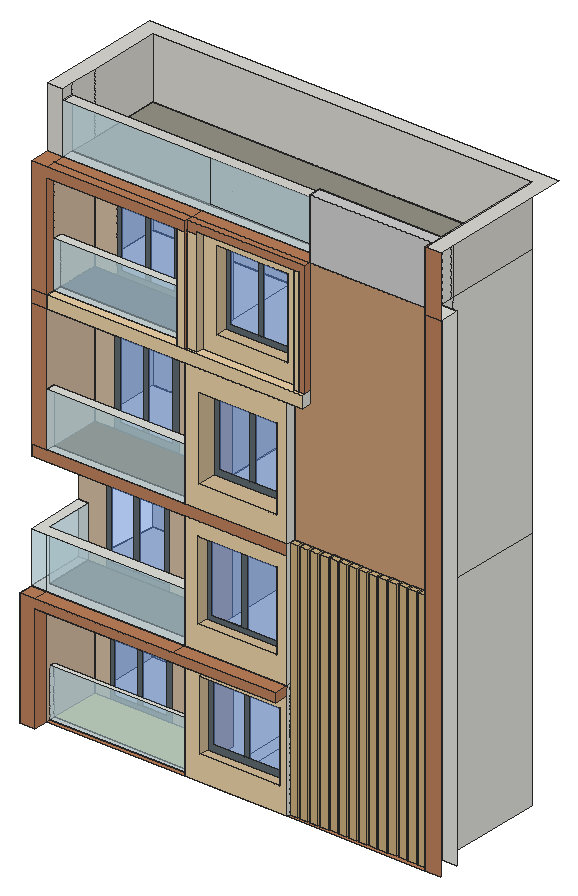
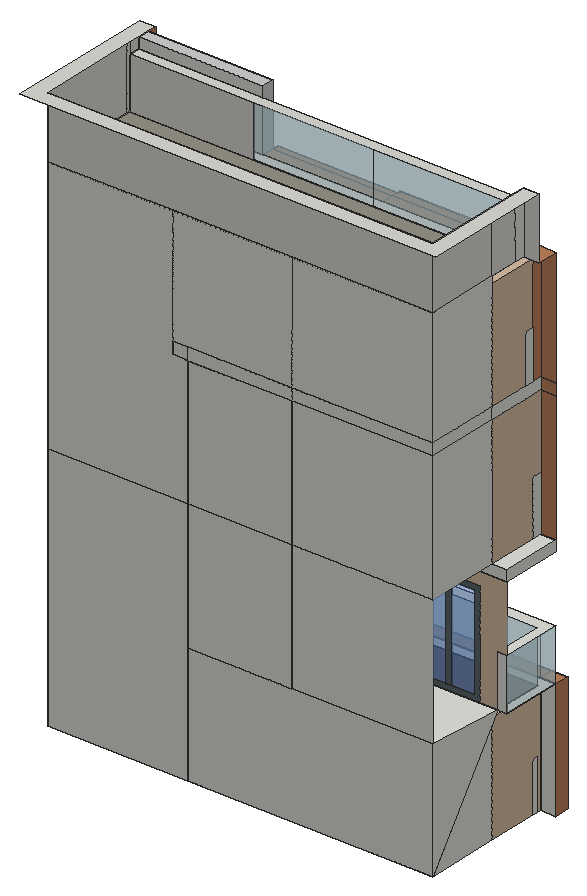
# SketchUp Ruby script. Lengths in inches.
U = 1.inch
M = Sketchup.active_model
def pt(a) = Geom::Point3d.new(a.map { |v| v * U })
def face(e, loops, mat)
  f = e.add_face(loops[0].map { |a| pt(a) })
  loops[1..].each { |l| e.add_face(l.map { |a| pt(a) }).erase! }
  f.material = f.back_material = mat if mat
  f
end
# faces: each face lists its corners as indices into pts; further lists are holes
def faces(e, pts, list, mat = nil) = list.each { |f| face(e, (f[0].is_a?(Array) ? f : [f]).map { |l| l.map { |i| pts[i] } }, mat) }
# xy, xz, yz: faces in a plane at the given z, y or x. An outline is a flat list of corners, or four numbers for a rectangle; further outlines are holes
def ring(l) = l.size == 4 ? [[l[0], l[1]], [l[2], l[1]], [l[2], l[3]], [l[0], l[3]]] : l.each_slice(2).to_a
def flat(e, list, mat, &to3) = list.each { |f| face(e, (f[0].is_a?(Array) ? f : [f]).map { |l| ring(l).map { |u, v| to3.(u, v) } }, mat) }
def xy(e, z, list, mat = nil) = flat(e, list, mat) { |x, y| [x, y, z] }
def xz(e, y, list, mat = nil) = flat(e, list, mat) { |x, z| [x, y, z] }
def yz(e, x, list, mat = nil) = flat(e, list, mat) { |y, z| [x, y, z] }
def lines(e, pts, list) = list.each { |a, b| e.add_line(pt(pts[a]), pt(pts[b])) }
# prism: a flat outline (further loops are holes) pulled along v
def prism(e, loops, v, mat = nil)
  f = face(e, loops, mat); d = Geom::Vector3d.new(v.map { |x| x * U })
  f.pushpull(f.normal.samedirection?(d) ? d.length : -d.length)
end
def box(e, o, s, mat = nil) = prism(e, [[o, [o[0] + s[0], o[1], o[2]], [o[0] + s[0], o[1] + s[1], o[2]], [o[0], o[1] + s[1], o[2]]]], [0, 0, s[2]], mat)
def at(x, y, z, deg = 0) = Geom::Transformation.translation(pt([x, y, z])) * Geom::Transformation.rotation(ORIGIN, Z_AXIS, deg.degrees)
def axes(o, x, y, z) = Geom::Transformation.new([*x, 0, *y, 0, *z, 0, *pt(o).to_a, 1])
def part(name) = M.definitions.add(name)
# library, detail: a bought-in or finely detailed component or shape, given as its bounding box
def library(name, o, s) = part(name).tap { |d| box(d.entities, o, s) }
def detail(e, o, s) = box(e.add_group.entities, o, s)
def put(e, d, t, mat = nil) = e.add_instance(d, t).tap { |i| i.material = mat if mat }
def group(e, t, mat = nil) = e.add_group.tap { |g| g.transformation = t; g.material = mat if mat }.entities
root = M.entities
M.materials.add("[Carpet Diamond Yellow]").color = [226, 217, 124]
M.materials.add("[Carrera Marble]").color = [207, 207, 207]
M.materials.add("[Cladding Siding Tan]").color = [201, 156, 118]
M.materials.add("[Formica Beige]").color = [237, 210, 167]
M.materials.add("[Formica Beige]1").color = [211, 187, 149]
M.materials.add("[Formica Graystone]").color = [149, 146, 135]
M.materials.add("[Formica Laminate Light]").color = [213, 189, 164]
M.materials.add("[Formica Speckled Grey]").color = [94, 105, 111]
M.materials.add("[Leather Blue]").color = [45, 57, 74]
M.materials.add("[Leather Red Brown]").color = [76, 40, 8]
M.materials.add("[Suede Dark Gray]").color = [85, 85, 85]
M.materials.add("[Terrazzo Tile Light]").color = [219, 217, 210]
M.materials.add("[Translucent Glass Blue]").color = [107, 160, 255]
M.materials["[Translucent Glass Blue]"].alpha = 0.5
M.materials.add("[Translucent Glass Safety]").color = [204, 235, 244]
M.materials["[Translucent Glass Safety]"].alpha = 0.5
M.materials.add("[Wood Floor Light]").color = [204, 176, 127]
M.materials.add("[Wood Veneer 02]").color = [190, 128, 91]
xy(root,194.875,[[145.12,201.25,161.99,201.25,161.99,326.6875,14.38,326.6875,14.38,257.75,145.12,257.75],[161.99,201.25,173.54,326.6875],[173.54,201.25,241.84,326.6875],[241.84,204.5,249.51,210.125],[251.46,204.5,259.13,210.125],
  [261.09,204.5,268.76,210.125],[270.59,204.5,278.26,210.125],[279.46,204.5,287.13,210.125],[288.4,204.5,296.07,210.125],[297.53,204.5,305.2,210.125],
  [306.71,204.5,314.38,210.125],[316.21,204.5,323.88,210.125],[325.53,204.5,333.2,210.125],[334.96,204.5,342.63,210.125],[344.46,204.5,352.13,210.125],
  [353.9,204.5,361.57,210.125],[363.28,204.5,370.95,210.125],[14.38,205.65,145.12,210.05]])
xy(root,194.875,[[14.38,210.05,145.12,257.75]],"[Carpet Diamond Yellow]")
xy(root,194.875,[[0,187.625,14.38,201.25],[14.38,201.25,145.12,205.65],[241.84,201.25,372.59,201.25,372.59,210.125,370.95,210.125,370.95,204.5,363.28,204.5,363.28,210.125,361.57,210.125,361.57,204.5,353.9,204.5,353.9,210.125,352.13,210.125,352.13,204.5,344.46,204.5,344.46,210.125,342.63,210.125,342.63,204.5,334.96,204.5,334.96,210.125,333.2,210.125,333.2,204.5,325.53,204.5,325.53,210.125,323.88,210.125,323.88,204.5,316.21,204.5,316.21,210.125,314.38,210.125,314.38,204.5,306.71,204.5,306.71,210.125,305.2,210.125,305.2,204.5,297.53,204.5,297.53,210.125,296.07,210.125,296.07,204.5,288.4,204.5,288.4,210.125,287.13,210.125,287.13,204.5,279.46,204.5,279.46,210.125,278.26,210.125,278.26,204.5,270.59,204.5,270.59,210.125,268.76,210.125,268.76,204.5,261.09,204.5,261.09,210.125,259.13,210.125,259.13,204.5,251.46,204.5,251.46,210.125,249.51,210.125,249.51,204.5,241.84,204.5]],"[Wood Veneer 02]")
xy(root,218.49,[[159.46,201.25,235.27,210.125]],"[Formica Beige]1")
xy(root,241.0625,[[14.38,205.65,145.12,210.05]])
xy(root,284.55,[[159.46,201.25,235.27,210.125]],"[Formica Beige]1")
xy(root,296.97,[[14.38,201.25,145.12,257.75]],"[Formica Laminate Light]")
xy(root,296.97,[[14.38,187.625,145.12,201.25],[145.12,187.625,241.84,201.25]],"[Wood Veneer 02]")
xy(root,305.25,[[0,201.25,0,257.75,8.76,257.75,8.76,211.77,145.12,211.77,145.12,201.25],[145.12,201.25,241.84,326.6875],[8.76,257.75,14.38,326.6875,145.12,326.6875,145.12,257.75]])
xy(root,305.25,[[8.76,211.77,145.12,257.75]],"[Suede Dark Gray]")
xy(root,305.25,[[0,187.625,14.38,201.25],[14.38,187.625,145.12,201.25],[145.12,187.625,241.84,201.25]],"[Wood Veneer 02]")
xy(root,327.94,[[157.85,201.25,232.54,211.6875]],"[Formica Beige]1")
xy(root,353.75,[[0,201.25,145.12,201.25,145.12,211.77,8.76,211.77,8.76,257.75,0,257.75]])
xy(root,402.63,[[157.85,201.25,232.54,211.6875]],"[Formica Beige]1")
xy(root,415.55,[[0,201.25,145.12,257.75]],"[Formica Laminate Light]")
xy(root,425.25,[[0,201.25,14.38,257.75],[14.38,201.25,145.12,210.125],[145.12,201.25,241.84,326.6875],[241.84,210.125,372.59,326.6875],[14.38,257.75,145.12,326.6875]])
xy(root,425.25,[[14.38,210.125,145.12,257.75]],"[Leather Red Brown]")
xy(root,425.25,[[241.84,204.5,249.51,210.125],[251.46,204.5,259.13,210.125],[261.09,204.5,268.76,210.125],[270.59,204.5,278.26,210.125],[279.46,204.5,287.13,210.125],
  [288.4,204.5,296.07,210.125],[297.53,204.5,305.2,210.125],[306.71,204.5,314.38,210.125],[316.21,204.5,323.88,210.125],[325.53,204.5,333.2,210.125],
  [334.96,204.5,342.63,210.125],[344.46,204.5,352.13,210.125],[353.9,204.5,361.57,210.125],[363.28,204.5,370.95,210.125]],"[Wood Floor Light]")
xy(root,446.97,[[158.21,201.25,232.27,219.625]],"[Formica Beige]1")
xy(root,476.75,[[14.38,201.25,145.12,210.125]])
xy(root,524.85,[[158.21,201.25,232.27,219.625]],"[Formica Beige]1")
xy(root,545.25,[[145.12,201.25,241.84,257.75],[241.84,210.125,256.71,257.75],[14.38,257.75,145.12,326.6875],[145.12,257.75,241.84,326.6875],[241.84,257.75,256.71,326.6875]])
xy(root,545.25,[[241.84,201.25,256.71,210.125]],"[Formica Beige]1")
xy(root,545.25,[[14.38,201.25,145.12,257.75]],"[Formica Laminate Light]")
xy(root,556.5,[[137.56,201.25,145.12,201.25,145.12,222.05,137.56,217.98],[145.12,203.8125,154.64,203.8125,154.64,210.125,241.84,210.125,241.84,222.05,145.12,222.05],[14.38,210.125,137.56,217.98],[241.84,210.125,256.71,222.05],[137.56,217.98,145.12,222.05,145.12,257.75,137.56,257.75],
  [145.12,222.05,241.84,326.6875],[241.84,222.05,256.71,326.6875],[14.38,257.75,145.12,326.6875]])
xy(root,556.5,[[14.38,201.25,137.56,210.125],[145.12,201.25,256.71,201.25,256.71,203.8125,245.875,203.8125,245.875,210.125,154.64,210.125,154.64,203.8125,145.12,203.8125]],"[Formica Beige]")
xy(root,556.5,[[14.38,217.98,137.56,257.75]],"[Leather Blue]")
xy(root,572.99,[[168.03,210.125,235.9,221.4375]],"[Formica Beige]1")
xy(root,601.25,[[14.38,210.125,137.56,217.98]])
xy(root,648.74,[[168.03,210.125,235.9,221.4375]],"[Formica Beige]1")
xy(root,655.84,[[14.38,201.25,137.56,210.125]])
xy(root,657.93,[[154.64,203.8125,245.875,210.125],[245.875,203.8125,251.36,210.125]])
xy(root,658.91,[[137.56,210.125,145.12,257.75]])
xy(root,658.91,[[14.38,210.125,137.56,257.75]],"[Formica Laminate Light]")
xy(root,665.25,[[372.59,201.25,386.97,220.875],[256.71,210.125,372.59,210.125,372.59,220.875,256.71,220.92],[372.59,220.875,256.71,220.92,145.12,220.96,14.38,221.01,14.38,231.4375,372.59,231.4375]])
xy(root,665.25,[[14.38,231.4375,372.59,326.6875]],"[Formica Graystone]")
xy(root,665.25,[[0,201.25,14.38,221.01],[14.38,201.25,145.12,210.125],[145.12,203.8125,256.71,210.125],[14.38,210.125,145.12,210.125,145.12,220.96,14.38,221.01],[145.12,210.125,256.71,210.125,256.71,220.92,145.12,220.96]],"[Wood Veneer 02]")
xy(root,712.875,[[372.59,220.875,372.59,231.4375,14.38,231.4375,14.38,221.01,256.71,220.92]],"[Terrazzo Tile Light]")
xy(root,722.875,[[256.71,210.125,372.59,210.125,372.59,220.875,256.71,220.92]],"[Carrera Marble]")
xy(root,722.875,[[372.59,201.25,386.97,201.25,386.97,341.07,0,341.07,0,221.01,14.38,221.01,14.38,326.6875,372.59,326.6875]],"[Terrazzo Tile Light]")
xz(root,187.625,[[0,194.875,14.38,194.875,14.38,296.97,241.84,296.97,241.84,305.25,0,305.25]],"[Wood Veneer 02]")
xz(root,201.25,[[0,194.875,0,305.25,241.84,305.25,241.84,296.97,14.38,296.97,14.38,194.875]])
xz(root,201.25,[[[145.12,194.875,241.84,296.97],[159.46,218.49,235.27,284.55]],[[145.12,305.25,241.84,415.55],[157.85,327.94,232.54,402.63]],[[145.12,425.25,241.84,545.25],[158.21,446.97,232.27,524.85]],[14.38,545.25,256.71,556.5],[137.56,556.5,145.12,655.84]],"[Formica Beige]")
xz(root,201.25,[[0,305.25,14.38,353.75],[14.38,305.25,145.12,353.75],[14.38,425.25,145.12,476.75]],"[Translucent Glass Safety]")
xz(root,201.25,[[372.59,194.875,386.97,665.25],[0,415.55,241.84,425.25],[0,425.25,14.38,545.25],[0,545.25,14.38,556.5],[0,556.5,14.38,556.5,14.38,655.84,145.12,655.84,145.12,665.25,0,665.25],
  [372.59,665.25,386.97,722.875]],"[Wood Veneer 02]")
xz(root,203.8125,[[145.12,556.5,154.64,655.84],[245.875,556.5,251.36,657.93]],"[Formica Beige]")
xz(root,203.8125,[[251.36,556.5,256.71,556.5,256.71,665.25,145.12,665.25,145.12,655.84,154.64,655.84,154.64,657.93,251.36,657.93]],"[Wood Veneer 02]")
xz(root,204.5,[[241.84,194.875,249.51,425.25],[251.46,194.875,259.13,425.25],[261.09,194.875,268.76,425.25],[270.59,194.875,278.26,425.25],[279.46,194.875,287.13,425.25],
  [288.4,194.875,296.07,425.25],[297.53,194.875,305.2,425.25],[306.71,194.875,314.38,425.25],[316.21,194.875,323.88,425.25],[325.53,194.875,333.2,425.25],
  [334.96,194.875,342.63,425.25],[344.46,194.875,352.13,425.25],[353.9,194.875,361.57,425.25],[363.28,194.875,370.95,425.25]],"[Wood Floor Light]")
xz(root,205.65,[[14.38,194.875,145.12,241.0625]],"[Translucent Glass Safety]")
xz(root,210.05,[[14.38,194.875,145.12,241.0625]],"[Translucent Glass Safety]")
xz(root,210.125,[[241.84,194.875,249.51,425.25],[249.51,194.875,251.46,425.25],[251.46,194.875,259.13,425.25],[259.13,194.875,261.09,425.25],[261.09,194.875,268.76,425.25],
  [268.76,194.875,270.59,425.25],[270.59,194.875,278.26,425.25],[278.26,194.875,279.46,425.25],[279.46,194.875,287.13,425.25],[287.13,194.875,288.4,425.25],
  [288.4,194.875,296.07,425.25],[296.07,194.875,297.53,425.25],[297.53,194.875,305.2,425.25],[305.2,194.875,306.71,425.25],[306.71,194.875,314.38,425.25],
  [314.38,194.875,316.21,425.25],[316.21,194.875,323.88,425.25],[323.88,194.875,325.53,425.25],[325.53,194.875,333.2,425.25],[333.2,194.875,334.96,425.25],
  [334.96,194.875,342.63,425.25],[342.63,194.875,344.46,425.25],[344.46,194.875,352.13,425.25],[352.13,194.875,353.9,425.25],[353.9,194.875,361.57,425.25],
  [361.57,194.875,363.28,425.25],[363.28,194.875,370.95,425.25],[370.95,194.875,372.59,425.25],[245.875,556.5,251.36,657.93],[14.38,655.84,137.56,658.91],
  [137.56,655.84,145.12,658.91]])
xz(root,210.125,[[256.71,665.25,372.59,722.875]],"[Carrera Marble]")
xz(root,210.125,[[241.84,425.25,372.59,425.25,372.59,665.25,256.71,665.25,256.71,545.25,241.84,545.25]],"[Cladding Siding Tan]")
xz(root,210.125,[[[154.64,556.5,245.875,657.93],[168.03,572.99,235.9,648.74]]],"[Formica Beige]")
xz(root,210.125,[[[159.46,218.49,235.27,284.55],[165.85,224.87,228.89,278.16]],[194.44,224.87,199.7,278.16]],"[Formica Speckled Grey]")
xz(root,210.125,[[165.85,224.87,194.44,278.16],[199.7,224.87,228.89,278.16]],"[Translucent Glass Blue]")
xz(root,210.125,[[14.38,425.25,145.12,476.75],[14.38,556.5,137.56,601.25]],"[Translucent Glass Safety]")
xz(root,211.6875,[[[157.85,327.94,232.54,402.63],[162.44,332.54,227.9375,398.03]],[190.96,332.54,196.83,398.03]],"[Formica Speckled Grey]")
xz(root,211.6875,[[162.44,332.54,190.96,398.03],[196.83,332.54,227.9375,398.03]],"[Translucent Glass Blue]")
xz(root,211.77,[[8.76,305.25,145.12,353.75]],"[Translucent Glass Safety]")
xz(root,217.98,[[14.38,556.5,137.56,601.25]],"[Translucent Glass Safety]")
xz(root,219.625,[[[158.21,446.97,232.27,524.85],[163.99,452.75,226.5,519.07]],[191.8,452.75,197.82,519.07]],"[Formica Speckled Grey]")
xz(root,219.625,[[163.99,452.75,191.8,519.07],[197.82,452.75,226.5,519.07]],"[Translucent Glass Blue]")
xz(root,220.875,[[372.59,194.875,386.97,665.25]])
xz(root,221.01,[[0,665.25,14.38,722.875]],"[Terrazzo Tile Light]")
xz(root,221.4375,[[[168.03,572.99,235.9,648.74],[172.92,577.88,231.01,643.85]],[198.96,577.88,204,643.85]],"[Formica Speckled Grey]")
xz(root,221.4375,[[172.92,577.88,198.96,643.85],[204,577.88,231.01,643.85]],"[Translucent Glass Blue]")
xz(root,231.4375,[[256.71,665.25,372.59,712.875]],"[Terrazzo Tile Light]")
xz(root,231.4375,[[14.38,665.25,145.12,712.875],[145.12,665.25,256.71,712.875]],"[Translucent Glass Safety]")
xz(root,257.75,[[14.38,296.97,145.12,296.97,145.12,305.25,8.76,305.25],[0,305.25,8.76,353.75],[0,415.55,145.12,425.25],[137.56,556.5,145.12,658.91]])
xz(root,257.75,[[14.38,194.875,29.51,194.875,29.51,289.4375,87.44,289.4375,87.44,194.875,145.12,194.875,145.12,296.97,14.38,296.97],[8.76,305.25,25.28,305.25,25.28,403.44,85.97,403.44,85.97,305.25,145.12,305.25,145.12,415.55,0,415.55,0,353.75,8.76,353.75],[14.38,425.25,32.41,425.25,32.41,522.5,95.03,522.5,95.03,425.25,145.12,425.25,145.12,545.25,14.38,545.25],[14.38,556.5,35.89,556.5,35.89,649.5625,95.45,649.5625,95.45,556.5,137.56,556.5,137.56,658.91,14.38,658.91]],"[Formica Laminate Light]")
xz(root,257.75,[[[29.51,194.875,87.44,289.4375],[34.01,199.38,82.9375,284.93]],[55.86,199.38,59.9,284.93],[[25.28,305.25,85.97,403.44],[30.6,310.57,80.64,398.12]],[51.99,310.57,57.07,398.12],[[32.41,425.25,95.03,522.5],[38.95,431.8,88.49,515.95]],
  [60.75,431.8,65.67,515.95],[[35.89,556.5,95.45,649.5625],[40.45,561.07,90.89,645]],[63.25,561.07,67.99,645]],"[Formica Speckled Grey]")
xz(root,257.75,[[34.01,199.38,55.86,284.93],[59.9,199.38,82.9375,284.93],[30.6,310.57,51.99,398.12],[57.07,310.57,80.64,398.12],[38.95,431.8,60.75,515.95],
  [65.67,431.8,88.49,515.95],[40.45,561.07,63.25,645],[67.99,561.07,90.89,645]],"[Translucent Glass Blue]")
xz(root,326.6875,[[14.38,194.875,241.84,305.25],[241.84,194.875,372.59,425.25],[14.38,305.25,145.12,425.25],[145.12,305.25,241.84,425.25],[14.38,425.25,145.12,545.25],
  [145.12,425.25,241.84,545.25],[241.84,425.25,372.59,425.25,372.59,665.25,256.71,665.25,256.71,545.25,241.84,545.25],[14.38,545.25,145.12,556.5],[145.12,545.25,241.84,556.5],[241.84,545.25,256.71,556.5],
  [14.38,556.5,145.12,665.25],[145.12,556.5,256.71,665.25]])
xz(root,326.6875,[[14.38,665.25,372.59,722.875]],"[Terrazzo Tile Light]")
yz(root,0,[[201.25,415.55,257.75,425.25]])
yz(root,0,[[201.25,305.25,257.75,353.75]],"[Translucent Glass Safety]")
yz(root,0,[[187.625,194.875,201.25,305.25]],"[Wood Veneer 02]")
yz(root,8.76,[[211.77,305.25,257.75,353.75]],"[Translucent Glass Safety]")
yz(root,14.38,[[205.65,194.875,210.05,241.0625],[257.75,194.875,326.6875,194.875,257.75,296.97],[201.25,425.25,210.125,476.75],[257.75,425.25,326.6875,545.25],[201.25,545.25,257.75,556.5],
  [257.75,545.25,326.6875,556.5],[210.125,556.5,217.98,601.25],[257.75,556.5,326.6875,665.25],[221.01,665.25,231.4375,712.875]])
yz(root,14.38,[[201.25,194.875,205.65,194.875,205.65,241.0625,210.05,241.0625,210.05,194.875,257.75,194.875,257.75,296.97,201.25,296.97],[210.125,425.25,257.75,425.25,257.75,545.25,201.25,545.25,201.25,476.75,210.125,476.75],[217.98,556.5,257.75,556.5,257.75,658.91,210.125,658.91,210.125,601.25,217.98,601.25]],"[Formica Laminate Light]")
yz(root,14.38,[[231.4375,665.25,257.75,722.875],[257.75,665.25,326.6875,722.875],[221.01,712.875,231.4375,722.875]],"[Terrazzo Tile Light]")
yz(root,14.38,[[187.625,194.875,201.25,296.97],[201.25,556.5,210.125,655.84]],"[Wood Veneer 02]")
yz(root,137.56,[[210.125,556.5,217.98,601.25]])
yz(root,137.56,[[201.25,556.5,201.25,655.84,210.125,655.84,210.125,658.91,257.75,658.91,257.75,556.5,217.98,556.5,217.98,601.25,210.125,601.25,210.125,556.5]],"[Formica Laminate Light]")
yz(root,145.12,[[205.65,194.875,210.05,241.0625],[201.25,305.25,211.77,353.75],[257.75,305.25,326.6875,425.25],[201.25,425.25,210.125,476.75],[257.75,425.25,326.6875,545.25],
  [203.8125,556.5,257.75,556.5,257.75,658.91,210.125,658.91,210.125,655.84,203.8125,655.84],[203.8125,655.84,210.125,658.91]])
yz(root,145.12,[[201.25,194.875,201.25,296.97,257.75,296.97,257.75,194.875,210.05,194.875,210.05,241.0625,205.65,241.0625,205.65,194.875],[211.77,305.25,211.77,353.75,201.25,353.75,201.25,415.55,257.75,415.55,257.75,305.25],[210.125,425.25,210.125,476.75,201.25,476.75,201.25,545.25,257.75,545.25,257.75,425.25]],"[Formica Laminate Light]")
yz(root,145.12,[[201.25,556.5,203.8125,665.25]],"[Wood Veneer 02]")
yz(root,154.64,[[203.8125,556.5,210.125,657.93]],"[Formica Beige]1")
yz(root,157.85,[[201.25,327.94,211.6875,402.63]],"[Formica Beige]1")
yz(root,158.21,[[201.25,446.97,219.625,524.85]],"[Formica Beige]1")
yz(root,159.46,[[201.25,218.49,210.125,284.55]],"[Formica Beige]1")
yz(root,168.03,[[210.125,572.99,221.4375,648.74]],"[Formica Beige]1")
yz(root,232.27,[[201.25,446.97,219.625,524.85]],"[Formica Beige]1")
yz(root,232.54,[[201.25,327.94,211.6875,402.63]],"[Formica Beige]1")
yz(root,235.27,[[201.25,218.49,210.125,284.55]],"[Formica Beige]1")
yz(root,235.9,[[210.125,572.99,221.4375,648.74]],"[Formica Beige]")
yz(root,241.84,[[201.25,194.875,204.5,305.25],[204.5,194.875,210.125,305.25],[210.125,194.875,326.6875,305.25],[201.25,305.25,204.5,425.25],[204.5,305.25,210.125,425.25],
  [210.125,305.25,326.6875,425.25],[201.25,425.25,210.125,545.25],[210.125,425.25,326.6875,545.25]])
yz(root,241.84,[[187.625,296.97,201.25,305.25]],"[Wood Veneer 02]")
yz(root,245.875,[[203.8125,556.5,210.125,657.93]],"[Formica Beige]")
yz(root,249.51,[[204.5,194.875,210.125,425.25]],"[Wood Floor Light]")
yz(root,251.36,[[203.8125,556.5,210.125,657.93]])
yz(root,251.46,[[204.5,194.875,210.125,305.25]])
yz(root,251.46,[[204.5,305.25,210.125,425.25]],"[Wood Floor Light]")
yz(root,256.71,[[201.25,545.25,210.125,556.5],[210.125,545.25,257.75,556.5],[257.75,545.25,326.6875,556.5]])
yz(root,256.71,[[210.125,665.25,220.92,722.875]],"[Carrera Marble]")
yz(root,256.71,[[203.8125,556.5,210.125,665.25]],"[Wood Veneer 02]")
yz(root,259.13,[[204.5,194.875,210.125,425.25]],"[Wood Floor Light]")
yz(root,261.09,[[204.5,194.875,210.125,305.25]])
yz(root,261.09,[[204.5,305.25,210.125,425.25]],"[Wood Floor Light]")
yz(root,268.76,[[204.5,194.875,210.125,425.25]],"[Wood Floor Light]")
yz(root,270.59,[[204.5,194.875,210.125,305.25]])
yz(root,270.59,[[204.5,305.25,210.125,425.25]],"[Wood Floor Light]")
yz(root,278.26,[[204.5,194.875,210.125,425.25]],"[Wood Floor Light]")
yz(root,279.46,[[204.5,194.875,210.125,305.25]])
yz(root,279.46,[[204.5,305.25,210.125,425.25]],"[Wood Floor Light]")
yz(root,287.13,[[204.5,194.875,210.125,425.25]],"[Wood Floor Light]")
yz(root,288.4,[[204.5,194.875,210.125,305.25]])
yz(root,288.4,[[204.5,305.25,210.125,425.25]],"[Wood Floor Light]")
yz(root,296.07,[[204.5,194.875,210.125,425.25]],"[Wood Floor Light]")
yz(root,297.53,[[204.5,194.875,210.125,305.25]])
yz(root,297.53,[[204.5,305.25,210.125,425.25]],"[Wood Floor Light]")
yz(root,305.2,[[204.5,194.875,210.125,425.25]],"[Wood Floor Light]")
yz(root,306.71,[[204.5,194.875,210.125,305.25]])
yz(root,306.71,[[204.5,305.25,210.125,425.25]],"[Wood Floor Light]")
yz(root,314.38,[[204.5,194.875,210.125,425.25]],"[Wood Floor Light]")
yz(root,316.21,[[204.5,194.875,210.125,305.25]])
yz(root,316.21,[[204.5,305.25,210.125,425.25]],"[Wood Floor Light]")
yz(root,323.88,[[204.5,194.875,210.125,425.25]],"[Wood Floor Light]")
yz(root,325.53,[[204.5,194.875,210.125,305.25]])
yz(root,325.53,[[204.5,305.25,210.125,425.25]],"[Wood Floor Light]")
yz(root,333.2,[[204.5,194.875,210.125,425.25]],"[Wood Floor Light]")
yz(root,334.96,[[204.5,194.875,210.125,305.25]])
yz(root,334.96,[[204.5,305.25,210.125,425.25]],"[Wood Floor Light]")
yz(root,342.63,[[204.5,194.875,210.125,425.25]],"[Wood Floor Light]")
yz(root,344.46,[[204.5,194.875,210.125,305.25]])
yz(root,344.46,[[204.5,305.25,210.125,425.25]],"[Wood Floor Light]")
yz(root,352.13,[[204.5,194.875,210.125,425.25]],"[Wood Floor Light]")
yz(root,353.9,[[204.5,194.875,210.125,305.25]])
yz(root,353.9,[[204.5,305.25,210.125,425.25]],"[Wood Floor Light]")
yz(root,361.57,[[204.5,194.875,210.125,425.25]],"[Wood Floor Light]")
yz(root,363.28,[[204.5,194.875,210.125,305.25]])
yz(root,363.28,[[204.5,305.25,210.125,425.25]],"[Wood Floor Light]")
yz(root,370.95,[[204.5,194.875,210.125,425.25]],"[Wood Floor Light]")
yz(root,372.59,[[220.875,194.875,234.35,425.25],[234.35,194.875,326.6875,425.25],[210.125,425.25,220.875,665.25],[220.875,425.25,234.35,665.25],[234.35,425.25,326.6875,665.25],
  [210.125,665.25,220.875,712.875],[220.875,665.25,231.4375,712.875],[210.125,712.875,220.875,722.875]])
yz(root,372.59,[[231.4375,665.25,234.35,722.875],[234.35,665.25,326.6875,722.875],[220.875,712.875,231.4375,722.875]],"[Terrazzo Tile Light]")
yz(root,372.59,[[201.25,194.875,210.125,665.25],[201.25,665.25,210.125,712.875],[201.25,712.875,210.125,722.875]],"[Wood Veneer 02]")
p = [[8.76,257.75,305.25],[14.38,257.75,296.97],[14.38,326.6875,194.875],[14.38,326.6875,305.25],[256.71,220.92,665.25],[256.71,220.92,712.875],
  [14.38,221.01,712.875],[14.38,221.01,665.25],[145.12,220.96,665.25],[372.59,220.875,665.25],[372.59,220.875,712.875],[372.59,220.875,722.875],
  [256.71,220.92,722.875],[256.71,257.75,556.5],[256.71,257.75,665.25],[145.12,257.75,658.91],[145.12,257.75,665.25]]
faces(root,p,[[0,1,2],[3,0,2],[9,4,5,10],[11,10,5,12]])
faces(root,p,[[4,5,6,7,8]],"[Translucent Glass Safety]")
lines(root,p,[[13,14],[15,16]])
